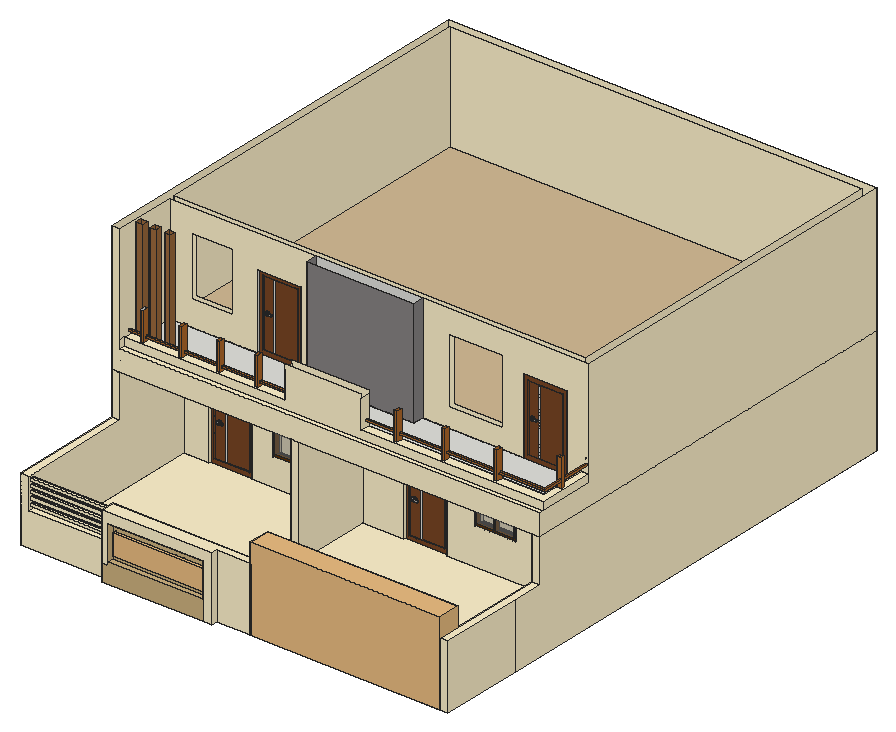
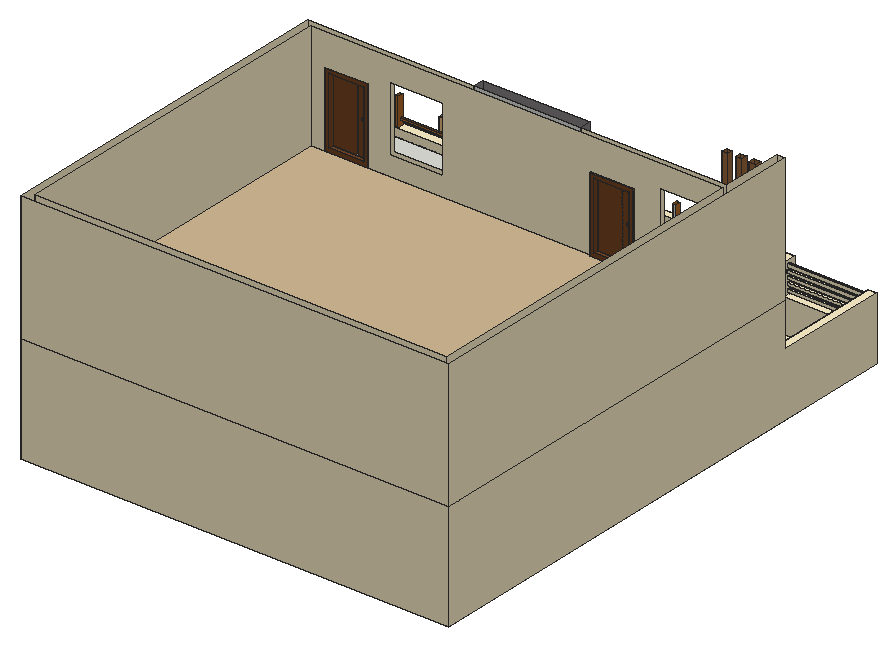
# SketchUp Ruby script. Lengths in inches.
U = 1.inch
M = Sketchup.active_model
def pt(a) = Geom::Point3d.new(a.map { |v| v * U })
def face(e, loops, mat)
  f = e.add_face(loops[0].map { |a| pt(a) })
  loops[1..].each { |l| e.add_face(l.map { |a| pt(a) }).erase! }
  f.material = f.back_material = mat if mat
  f
end
# faces: each face lists its corners as indices into pts; further lists are holes
def faces(e, pts, list, mat = nil) = list.each { |f| face(e, (f[0].is_a?(Array) ? f : [f]).map { |l| l.map { |i| pts[i] } }, mat) }
# xy, xz, yz: faces in a plane at the given z, y or x. An outline is a flat list of corners, or four numbers for a rectangle; further outlines are holes
def ring(l) = l.size == 4 ? [[l[0], l[1]], [l[2], l[1]], [l[2], l[3]], [l[0], l[3]]] : l.each_slice(2).to_a
def flat(e, list, mat, &to3) = list.each { |f| face(e, (f[0].is_a?(Array) ? f : [f]).map { |l| ring(l).map { |u, v| to3.(u, v) } }, mat) }
def xy(e, z, list, mat = nil) = flat(e, list, mat) { |x, y| [x, y, z] }
def xz(e, y, list, mat = nil) = flat(e, list, mat) { |x, z| [x, y, z] }
def yz(e, x, list, mat = nil) = flat(e, list, mat) { |y, z| [x, y, z] }
def lines(e, pts, list) = list.each { |a, b| e.add_line(pt(pts[a]), pt(pts[b])) }
# prism: a flat outline (further loops are holes) pulled along v
def prism(e, loops, v, mat = nil)
  f = face(e, loops, mat); d = Geom::Vector3d.new(v.map { |x| x * U })
  f.pushpull(f.normal.samedirection?(d) ? d.length : -d.length)
end
def box(e, o, s, mat = nil) = prism(e, [[o, [o[0] + s[0], o[1], o[2]], [o[0] + s[0], o[1] + s[1], o[2]], [o[0], o[1] + s[1], o[2]]]], [0, 0, s[2]], mat)
def at(x, y, z, deg = 0) = Geom::Transformation.translation(pt([x, y, z])) * Geom::Transformation.rotation(ORIGIN, Z_AXIS, deg.degrees)
def axes(o, x, y, z) = Geom::Transformation.new([*x, 0, *y, 0, *z, 0, *pt(o).to_a, 1])
def part(name) = M.definitions.add(name)
# library, detail: a bought-in or finely detailed component or shape, given as its bounding box
def library(name, o, s) = part(name).tap { |d| box(d.entities, o, s) }
def detail(e, o, s) = box(e.add_group.entities, o, s)
def put(e, d, t, mat = nil) = e.add_instance(d, t).tap { |i| i.material = mat if mat }
def group(e, t, mat = nil) = e.add_group.tap { |g| g.transformation = t; g.material = mat if mat }.entities
root = M.entities
M.materials.add("[Aluminum]").color = [179, 179, 179]
M.materials.add("[Brick Tumbled]").color = [135, 132, 132]
M.materials.add("[Color C08]").color = [102, 51, 0]
M.materials.add("[Color D01]").color = [255, 242, 204]
M.materials.add("[Formica Beige]").color = [211, 187, 149]
M.materials.add("[Stone Sandstone Ashlar Light]").color = [206, 178, 128]
M.materials.add("[Translucent Glass Gray]").color = [128, 128, 128]
M.materials["[Translucent Glass Gray]"].alpha = 0.5
M.materials.add("[Wood Bamboo]").color = [177, 105, 43]
M.materials.add("[Wood Floor]").color = [155, 105, 61]
M.materials.add("[Wood Veneer 01]").color = [120, 70, 37]
c1 = library("Wrought-iron gates",[-30,-13,0],[261.35,24.4,62.45])
c2 = part("Group\#1")
xy(c2.entities,0,[[0,1.5625,48,2.9375],[0,2.9375,48,11.9375]],"[Wood Veneer 01]")
xy(c2.entities,4.26,[[4.26,1.5625,43.74,2.9375],[4.26,2.9375,43.74,11.9375]],"[Wood Veneer 01]")
xy(c2.entities,41.66,[[8.83,0,8.83,1.4375,9.58,1.4375,9.58,0.72,15.08,0.72,15.08,0]],"[Aluminum]")
xy(c2.entities,43.35,[[8.83,0,15.08,0,15.08,0.72,9.58,0.72,9.58,1.4375,8.83,1.4375]],"[Aluminum]")
xy(c2.entities,79.74,[[4.26,1.5625,16.16,2.9375],[16.16,1.5625,16.99,2.9375],[16.99,1.5625,43.74,2.9375],[4.26,2.9375,43.74,11.9375]],"[Wood Veneer 01]")
xy(c2.entities,84,[[0,1.5625,48,2.9375],[0,2.9375,48,11.9375]],"[Wood Veneer 01]")
xz(c2.entities,0,[[8.83,41.66,15.08,43.35]],"[Aluminum]")
xz(c2.entities,0.72,[[9.58,41.66,15.08,43.35]],"[Aluminum]")
xz(c2.entities,1.4375,[[[9.24,40.44,9.77,40.51,10.27,40.72,10.7,41.05,11.03,41.47,11.23,41.97,11.3,42.5,11.23,43.04,11.03,43.54,10.7,43.96,10.27,44.29,9.77,44.5,9.24,44.57,8.71,44.5,8.21,44.29,7.78,43.96,7.45,43.54,7.25,43.04,7.18,42.5,7.25,41.97,7.45,41.47,7.78,41.05,8.21,40.72,8.71,40.51],[8.83,41.66,9.58,43.35]]],"[Aluminum]")
xz(c2.entities,1.5625,[[[0,0,48,84],[4.26,4.26,43.74,79.74]]],"[Wood Veneer 01]")
xz(c2.entities,2.9375,[[[0,0,48,84],[4.26,4.26,43.74,79.74]],[16.16,4.26,16.99,79.74]])
xz(c2.entities,2.9375,[[[4.26,4.26,16.16,79.74],[9.24,40.44,8.71,40.51,8.21,40.72,7.78,41.05,7.45,41.47,7.25,41.97,7.18,42.5,7.25,43.04,7.45,43.54,7.78,43.96,8.21,44.29,8.71,44.5,9.24,44.57,9.77,44.5,10.27,44.29,10.7,43.96,11.03,43.54,11.23,43.04,11.3,42.5,11.23,41.97,11.03,41.47,10.7,41.05,10.27,40.72,9.77,40.51]],[16.99,4.26,43.74,79.74]],"[Wood Veneer 01]")
xz(c2.entities,11.9375,[[[0,0,48,84],[4.26,4.26,43.74,79.74]]],"[Wood Veneer 01]")
yz(c2.entities,0,[[1.5625,0,2.9375,84],[2.9375,0,11.9375,84]],"[Wood Veneer 01]")
yz(c2.entities,4.26,[[1.5625,4.26,2.9375,79.74],[2.9375,4.26,11.9375,79.74]],"[Wood Veneer 01]")
yz(c2.entities,8.83,[[0,41.66,1.4375,43.35]],"[Aluminum]")
yz(c2.entities,9.58,[[0.72,41.66,1.4375,43.35]],"[Aluminum]")
yz(c2.entities,15.08,[[0,41.66,0.72,43.35]],"[Aluminum]")
yz(c2.entities,43.74,[[1.5625,4.26,2.9375,79.74],[2.9375,4.26,11.9375,79.74]],"[Wood Veneer 01]")
yz(c2.entities,48,[[1.5625,0,2.9375,84],[2.9375,0,11.9375,84]],"[Wood Veneer 01]")
p = [[8.71,2.9375,40.51],[9.24,2.9375,40.44],[9.24,1.4375,40.44],[8.71,1.4375,40.51],[9.77,2.9375,40.51],[9.77,1.4375,40.51],
  [8.21,2.9375,40.72],[8.21,1.4375,40.72],[10.27,2.9375,40.72],[10.27,1.4375,40.72],[7.78,2.9375,41.05],[7.78,1.4375,41.05],
  [10.7,2.9375,41.05],[10.7,1.4375,41.05],[7.45,2.9375,41.47],[7.45,1.4375,41.47],[11.03,2.9375,41.47],[11.03,1.4375,41.47],
  [7.25,2.9375,41.97],[7.25,1.4375,41.97],[11.23,2.9375,41.97],[11.23,1.4375,41.97],[7.18,2.9375,42.5],[7.18,1.4375,42.5],
  [11.3,2.9375,42.5],[11.3,1.4375,42.5],[7.25,2.9375,43.04],[7.25,1.4375,43.04],[11.23,2.9375,43.04],[11.23,1.4375,43.04],
  [7.45,2.9375,43.54],[7.45,1.4375,43.54],[11.03,2.9375,43.54],[11.03,1.4375,43.54],[7.78,2.9375,43.96],[7.78,1.4375,43.96],
  [10.7,2.9375,43.96],[10.7,1.4375,43.96],[8.21,2.9375,44.29],[8.21,1.4375,44.29],[10.27,2.9375,44.29],[10.27,1.4375,44.29],
  [8.71,2.9375,44.5],[8.71,1.4375,44.5],[9.77,2.9375,44.5],[9.77,1.4375,44.5],[9.24,2.9375,44.57],[9.24,1.4375,44.57]]
faces(c2.entities,p,[[0,1,2,3],[1,4,5,2],[6,0,3,7],[4,8,9,5],[10,6,7,11],[8,12,13,9],[14,10,11,15],[12,16,17,13],
  [18,14,15,19],[16,20,21,17],[22,18,19,23],[20,24,25,21],[26,22,23,27],[24,28,29,25],[30,26,27,31],[28,32,33,29],
  [34,30,31,35],[32,36,37,33],[38,34,35,39],[36,40,41,37],[42,38,39,43],[40,44,45,41],[46,42,43,47],[44,46,47,45]],"[Aluminum]")
c3 = library("RAMA",[0.59,0,0],[102.88,23.44,4])
c4 = part("Group\#4")
xy(c4.entities,0,[[0,0,52.875,9]],"[Color C08]")
xy(c4.entities,2.31,[[2.31,0,24.96,9],[26.98,0,50.56,9]],"[Color C08]")
xy(c4.entities,50.56,[[2.31,0,24.96,9],[26.98,0,50.56,9]],"[Color C08]")
xy(c4.entities,52.875,[[0,0,52.875,9]],"[Color C08]")
xz(c4.entities,0,[[[0,0,52.875,52.875],[26.98,2.31,50.56,50.56],[2.31,2.31,24.96,50.56]]],"[Color C08]")
xz(c4.entities,0,[[2.31,2.31,24.96,50.56],[26.98,2.31,50.56,50.56]],"[Translucent Glass Gray]")
xz(c4.entities,9,[[[0,0,52.875,52.875],[26.98,2.31,50.56,50.56],[2.31,2.31,24.96,50.56]]],"[Color C08]")
yz(c4.entities,0,[[0,0,9,52.875]],"[Color C08]")
yz(c4.entities,2.31,[[0,2.31,9,50.56]],"[Color C08]")
yz(c4.entities,24.96,[[0,2.31,9,50.56]],"[Color C08]")
yz(c4.entities,26.98,[[0,2.31,9,50.56]],"[Color C08]")
yz(c4.entities,50.56,[[0,2.31,9,50.56]],"[Color C08]")
yz(c4.entities,52.875,[[0,0,9,52.875]],"[Color C08]")
xy(root,0,[[96.6875,0,210.23,6.75],[210.23,0,220.17,6.75],[258.29,6.75,471,15.75],[9,15.75,471,15.75,471,225.0625,303.9375,225.0625,303.9375,235.3125,255.9375,235.3125,255.9375,225.0625,209.375,225.0625,209.375,135.4,200.375,135.4,200.375,225.0625,85.29,225.0625,85.29,235.3125,200.375,235.3125,200.375,597.75,9,597.75,9,235.3125,37.29,235.3125,37.29,225.0625,9,225.0625],[0,101.375,0,606.75,480,606.75,480,101.375,471,101.375,471,225.0625,303.9375,225.0625,303.9375,235.3125,471,235.3125,471,597.75,9,597.75,9,235.3125,37.29,235.3125,37.29,225.0625,9,225.0625,9,101.375],
  [200.375,135.4,209.375,235.3125],[85.29,225.0625,85.29,235.3125,200.375,235.3125,200.375,314.26,209.375,314.26,209.375,235.3125,200.375,235.3125,200.375,225.0625],[209.375,225.0625,255.9375,235.3125],[209.375,235.3125,471,235.3125,471,597.75,209.375,597.75,209.375,383.08,200.375,383.08,200.375,314.26,209.375,314.26],[200.375,383.08,209.375,597.75]],"[Color D01]")
xy(root,22.14,[[104,0,210.23,6.75]],"[Stone Sandstone Ashlar Light]")
xy(root,30.78,[[109.26,225.0625,164.32,235.3125]],"[Color D01]")
xy(root,37.75,[[9,6.75,96.6875,15.75]],"[Color D01]")
xy(root,40.97,[[9,8.99,96.6875,11.93]],"[Color D01]")
xy(root,41.23,[[335.7,225.0625,380.95,235.3125]],"[Color D01]")
xy(root,44.41,[[9,8.99,96.6875,11.93]],"[Color D01]")
xy(root,47.79,[[9,8.99,96.9375,11.93]],"[Color D01]")
xy(root,51.22,[[9,8.99,96.9375,11.93]],"[Color D01]")
xy(root,53.97,[[9,8.99,96.6875,11.93]],"[Color D01]")
xy(root,57.41,[[9,8.99,96.6875,11.93]],"[Color D01]")
xy(root,60.1,[[9,8.99,96,11.93]],"[Color D01]")
xy(root,61.125,[[104,0,210.23,6.75]],"[Stone Sandstone Ashlar Light]")
xy(root,63.54,[[9,8.99,96,11.93]],"[Color D01]")
xy(root,66.35,[[9,8.99,97.4375,11.93]],"[Color D01]")
xy(root,69.79,[[9,8.99,97.4375,11.93]],"[Color D01]")
xy(root,72,[[96.6875,0,220.17,0,220.17,6.75,258.29,6.75,258.29,15.75,96.6875,15.75],[0,6.75,9,135.4],[471,6.75,480,135.4]],"[Color D01]")
xy(root,84,[[37.29,225.0625,85.29,235.3125],[255.9375,225.0625,303.9375,235.3125]],"[Color D01]")
xy(root,94.1,[[335.7,225.0625,380.95,235.3125]],"[Color D01]")
xy(root,98.875,[[200.375,314.26,209.375,383.08]],"[Color D01]")
xy(root,102.59,[[109.26,225.0625,164.32,235.3125]],"[Color D01]")
xy(root,120,[[0,135.4,480,606.75]])
xy(root,120,[[0,135.4,9,135.4,9,225.0625,200.375,225.0625,200.375,135.4,209.375,135.4,209.375,597.75,200.375,597.75,200.375,235.3125,9,235.3125,9,597.75,471,597.75,471,235.3125,209.375,235.3125,209.375,225.0625,471,225.0625,471,135.4,480,135.4,480,606.75,0,606.75],[9,235.3125,200.375,597.75],[209.375,235.3125,471,597.75]],"[Color D01]")
xy(root,133,[[9,151.78,9,204.4,108.75,204.4,108.75,210.4,156.75,210.4,156.75,204.4,172.75,204.4,172.75,192.4,292.75,192.4,292.75,204.4,407.0625,204.4,407.0625,210.4,455.0625,210.4,455.0625,204.4,471,204.4,471,151.78]])
xy(root,143.9375,[[9,140.9,9,151.78,471,151.78,471,204.4,480,204.4,480,140.9],[[9,151.78,471,151.78,471,204.4,455.0625,204.4,455.0625,210.4,407.0625,210.4,407.0625,204.4,292.75,204.4,292.75,192.4,172.75,192.4,172.75,204.4,156.75,204.4,156.75,210.4,108.75,210.4,108.75,204.4,9,204.4],[11.75,154.17,19.6875,160.61],[27.8125,154.17,35,160.61],[43.5625,154.17,50.1875,160.61]],[172.75,192.4,292.75,204.4],[156.75,204.4,407.0625,210.4]])
xy(root,143.9375,[[9,135.4,480,140.9]],"[Color D01]")
xy(root,143.9375,[[9,210.4,471,597.75]],"[Formica Beige]")
xy(root,152.9375,[[[9,140.9,188.91,151.78],[25.45,143.88,28.82,150.13],[68.13,143.88,71.51,150.13],[110.26,143.88,113.63,150.13],[152.95,143.88,156.32,150.13]],[[274.98,140.9,480,140.9,480,204.4,471,204.4,471,151.78,274.98,151.78],[309.7,143.88,313.07,150.13],[362.95,143.88,366.32,150.13],[421.51,143.88,424.88,150.13],[472.3125,168.86,477.25,172.24]]],"[Color D01]")
xy(root,157.15,[[9,146.22,28.82,148.34]])
xy(root,157.15,[[28.82,146.22,188.91,148.34]],"[Wood Bamboo]")
xy(root,159.27,[[9,146.22,28.82,148.34],[28.82,146.22,188.91,148.34]],"[Wood Bamboo]")
xy(root,160.11,[[274.98,145.89,274.98,148.02,475.1875,148.02,475.1875,207.71,477.01,207.71,477.01,145.89]],"[Wood Bamboo]")
xz(root,0,[[210.23,0,220.17,0,220.17,72,96.6875,72,96.6875,18.4375,104,18.4375,104,61.125,210.23,61.125]],"[Color D01]")
xz(root,0,[[96.6875,0,210.23,0,210.23,22.14,104,22.14,104,18.4375,96.6875,18.4375]],"[Stone Sandstone Ashlar Light]")
xz(root,6.75,[[0,0,96.6875,0,96.6875,37.75,9,37.75,9,72,0,72],[220.17,0,258.29,0,258.29,72,220.25,72,220.25,61.125,220.17,61.125],[471,0,480,72],[220.17,61.125,220.25,72]],"[Color D01]")
xz(root,6.75,[[104,22.14,210.23,61.125]],"[Stone Sandstone Ashlar Light]")
xz(root,8.99,[[9,40.97,96.6875,44.41],[9,47.79,96.9375,51.22],[9,53.97,96.6875,57.41],[9,60.1,96,63.54],[9,66.35,97.4375,69.79]],"[Color D01]")
xz(root,11.93,[[9,40.97,96.6875,44.41],[9,47.79,96.9375,51.22],[9,53.97,96.6875,57.41],[9,60.1,96,63.54],[9,66.35,97.4375,69.79]],"[Color D01]")
xz(root,15.75,[[9,0,9,37.75,96.6875,37.75,96.6875,72,258.29,72,258.29,0]],"[Color D01]")
xz(root,135.4,[[200.375,0,209.375,120],[0,72,9,120],[471,72,480,120],[0,120,480,120,480,143.9375,9,143.9375,9,263.9375,0,263.9375]],"[Color D01]")
xz(root,140.9,[[9,143.9375,480,143.9375,480,152.9375,274.98,152.9375,274.98,188.9375,188.91,188.9375,188.91,152.9375,9,152.9375]],"[Color D01]")
xz(root,143.88,[[25.45,152.9375,28.82,185],[68.13,152.9375,71.51,184.18],[110.26,152.9375,113.63,184.18],[152.95,152.9375,156.32,184.4375],[309.7,152.9375,313.07,184],
  [362.95,152.9375,366.32,184.5625],[421.51,152.9375,424.88,184.18]],"[Wood Bamboo]")
xz(root,145.89,[[274.98,160.11,477.01,162.24]],"[Wood Bamboo]")
xz(root,146.22,[[9,157.15,28.82,159.27],[28.82,157.15,188.91,159.27]],"[Wood Bamboo]")
xz(root,148.02,[[274.98,160.11,475.1875,162.24]],"[Wood Bamboo]")
xz(root,148.34,[[9,157.15,28.82,159.27],[28.82,157.15,188.91,159.27]],"[Wood Bamboo]")
xz(root,150.13,[[110.26,152.9375,113.63,184.18],[152.95,152.9375,156.32,184.4375]])
xz(root,150.13,[[25.45,152.9375,28.82,185],[68.13,152.9375,71.51,184.18],[309.7,152.9375,313.07,184],[362.95,152.9375,366.32,184.5625],[421.51,152.9375,424.88,184.18]],"[Wood Bamboo]")
xz(root,151.78,[[9,133,471,143.9375]])
xz(root,151.78,[[9,143.9375,9,152.9375,188.91,152.9375,188.91,188.9375,274.98,188.9375,274.98,152.9375,471,152.9375,471,143.9375]],"[Color D01]")
xz(root,154.17,[[11.75,143.9375,19.6875,263.9375],[27.8125,143.9375,35,263.9375],[43.5625,143.9375,50.1875,263.9375]],"[Wood Floor]")
xz(root,160.61,[[11.75,143.9375,19.6875,263.9375],[27.8125,143.9375,35,263.9375],[43.5625,143.9375,50.1875,263.9375]],"[Wood Floor]")
xz(root,168.86,[[472.3125,152.9375,477.25,184.1875]],"[Wood Bamboo]")
xz(root,172.24,[[472.3125,152.9375,477.25,184.1875]],"[Wood Bamboo]")
xz(root,192.4,[[172.75,133,292.75,143.9375]])
xz(root,192.4,[[172.75,143.9375,292.75,263.9375]],"[Brick Tumbled]")
xz(root,204.4,[[9,133,108.75,143.9375],[156.75,133,172.75,143.9375],[292.75,133,407.0625,143.9375],[455.0625,133,471,143.9375],[172.75,143.9375,292.75,263.9375],
  [471,143.9375,480,152.9375]])
xz(root,204.4,[[[9,143.9375,108.75,143.9375,108.75,227.9375,156.75,227.9375,156.75,143.9375,172.75,143.9375,172.75,263.9375,9,263.9375],[33.82,172.75,80.13,238.56]],[[292.75,143.9375,407.0625,143.9375,407.0625,227.9375,455.0625,227.9375,455.0625,143.9375,471,143.9375,471,152.9375,480,152.9375,480,263.9375,292.75,263.9375],[322.9,165.73,382.78,238.86],[475.1875,166.24,477.01,168.36]]],"[Color D01]")
xz(root,207.71,[[475.1875,160.11,477.01,162.24]])
xz(root,210.4,[[108.75,133,156.75,143.9375],[407.0625,133,455.0625,143.9375]])
xz(root,210.4,[[[9,143.9375,9,263.9375,471,263.9375,471,143.9375,455.0625,143.9375,455.0625,227.9375,407.0625,227.9375,407.0625,143.9375,156.75,143.9375,156.75,227.9375,108.75,227.9375,108.75,143.9375],[322.9,165.73,382.78,238.86],[33.82,172.75,80.13,238.56]]],"[Color D01]")
xz(root,225.0625,[[[9,0,37.29,0,37.29,84,85.29,84,85.29,0,200.375,0,200.375,120,9,120],[109.26,30.78,164.32,102.59]],[[209.375,0,255.9375,0,255.9375,84,303.9375,84,303.9375,0,471,0,471,120,209.375,120],[335.7,41.23,380.95,94.1]]],"[Color D01]")
xz(root,235.3125,[[[9,0,9,120,200.375,120,200.375,0,85.29,0,85.29,84,37.29,84,37.29,0],[109.26,30.78,164.32,102.59]],[[209.375,0,209.375,120,471,120,471,0,303.9375,0,303.9375,84,255.9375,84,255.9375,0],[335.7,41.23,380.95,94.1]]],"[Color D01]")
xz(root,314.26,[[200.375,0,209.375,98.875]],"[Color D01]")
xz(root,383.08,[[200.375,0,209.375,98.875]],"[Color D01]")
xz(root,597.75,[[9,0,200.375,120],[200.375,0,209.375,120],[209.375,0,471,120],[9,143.9375,471,263.9375]],"[Color D01]")
xz(root,606.75,[[0,0,480,120],[0,120,480,263.9375]],"[Color D01]")
yz(root,0,[[6.75,0,6.75,72,135.4,72,135.4,120,606.75,120,606.75,0],[135.4,120,606.75,263.9375]],"[Color D01]")
yz(root,9,[[151.78,133,204.4,143.9375],[140.9,143.9375,151.78,152.9375]])
yz(root,9,[[[15.75,0,225.0625,0,225.0625,120,135.4,120,135.4,72,6.75,72,6.75,37.75,15.75,37.75],[8.99,40.97,11.93,44.41],[8.99,47.79,11.93,51.22],[8.99,53.97,11.93,57.41],[8.99,60.1,11.93,63.54],[8.99,66.35,11.93,69.79]],[235.3125,0,597.75,120],[135.4,143.9375,140.9,152.9375],[[151.78,143.9375,204.4,143.9375,204.4,263.9375,135.4,263.9375,135.4,152.9375,151.78,152.9375],[146.02,178.55,148.14,180.67],[146.02,171.67,148.14,173.8],[146.02,164.48,148.14,166.61],[146.22,157.15,148.34,159.27]],[210.4,143.9375,597.75,263.9375]],"[Color D01]")
yz(root,11.75,[[154.17,143.9375,160.61,263.9375]],"[Wood Floor]")
yz(root,19.6875,[[154.17,143.9375,160.61,263.9375]],"[Wood Floor]")
yz(root,25.45,[[143.88,152.9375,150.13,185]])
yz(root,27.8125,[[154.17,143.9375,160.61,263.9375]],"[Wood Floor]")
yz(root,28.82,[[146.22,157.15,148.34,159.27]])
yz(root,28.82,[[[143.88,152.9375,150.13,185],[146.02,178.55,148.14,180.67],[146.02,171.67,148.14,173.8],[146.02,164.48,148.14,166.61],[146.22,157.15,148.34,159.27]]],"[Wood Bamboo]")
yz(root,35,[[154.17,143.9375,160.61,263.9375]],"[Wood Floor]")
yz(root,37.29,[[225.0625,0,235.3125,84]],"[Color D01]")
yz(root,43.5625,[[154.17,143.9375,160.61,263.9375]],"[Wood Floor]")
yz(root,50.1875,[[154.17,143.9375,160.61,263.9375]],"[Wood Floor]")
yz(root,68.13,[[143.88,152.9375,150.13,184.18]],"[Wood Bamboo]")
yz(root,71.51,[[143.88,152.9375,150.13,184.18]],"[Wood Bamboo]")
yz(root,85.29,[[225.0625,0,235.3125,84]],"[Color D01]")
yz(root,96,[[8.99,60.1,11.93,63.54]],"[Color D01]")
yz(root,96.6875,[[[0,0,0,72,15.75,72,15.75,37.75,6.75,37.75,6.75,0],[8.99,40.97,11.93,44.41],[8.99,53.97,11.93,57.41]]],"[Color D01]")
yz(root,96.9375,[[8.99,47.79,11.93,51.22]],"[Color D01]")
yz(root,97.4375,[[8.99,66.35,11.93,69.79]],"[Color D01]")
yz(root,104,[[0,22.14,6.75,61.125]],"[Stone Sandstone Ashlar Light]")
yz(root,108.75,[[204.4,133,210.4,143.9375],[204.4,143.9375,210.4,227.9375]])
yz(root,109.26,[[225.0625,30.78,235.3125,102.59]],"[Color D01]")
yz(root,110.26,[[143.88,152.9375,150.13,184.18]],"[Wood Bamboo]")
yz(root,113.63,[[143.88,152.9375,150.13,184.18]],"[Wood Bamboo]")
yz(root,152.95,[[143.88,152.9375,150.13,184.4375]],"[Wood Bamboo]")
yz(root,156.32,[[143.88,152.9375,150.13,184.4375]],"[Wood Bamboo]")
yz(root,156.75,[[204.4,133,210.4,143.9375],[204.4,143.9375,210.4,227.9375]])
yz(root,164.32,[[225.0625,30.78,235.3125,102.59]],"[Color D01]")
yz(root,172.75,[[192.4,133,204.4,143.9375]])
yz(root,172.75,[[192.4,143.9375,204.4,263.9375]],"[Brick Tumbled]")
yz(root,188.91,[[[140.9,152.9375,151.78,184.18],[146.22,157.15,148.34,159.27]]],"[Color D01]")
yz(root,200.375,[[135.4,0,225.0625,120],[235.3125,0,235.3125,120,597.75,120,597.75,0,383.08,0,383.08,98.875,314.26,98.875,314.26,0]],"[Color D01]")
yz(root,209.375,[[135.4,0,225.0625,120],[225.0625,0,235.3125,120],[235.3125,0,314.26,0,314.26,98.875,383.08,98.875,383.08,0,597.75,0,597.75,120,235.3125,120]],"[Color D01]")
yz(root,210.23,[[0,22.14,6.75,61.125]],"[Stone Sandstone Ashlar Light]")
yz(root,220.17,[[0,0,6.75,72]],"[Color D01]")
yz(root,255.9375,[[225.0625,0,235.3125,84]],"[Color D01]")
yz(root,258.29,[[6.75,0,15.75,72]],"[Color D01]")
yz(root,274.98,[[[140.9,152.9375,151.78,184.18],[145.89,177.99,148.02,180.49],[145.89,172.43,148.02,174.55],[145.89,166.24,148.02,168.36],[145.89,160.11,148.02,162.24]]],"[Color D01]")
yz(root,292.75,[[192.4,133,204.4,143.9375]])
yz(root,292.75,[[192.4,143.9375,204.4,263.9375]],"[Brick Tumbled]")
yz(root,303.9375,[[225.0625,0,235.3125,84]],"[Color D01]")
yz(root,309.7,[[143.88,152.9375,150.13,184]],"[Wood Bamboo]")
yz(root,313.07,[[143.88,152.9375,150.13,184]],"[Wood Bamboo]")
yz(root,335.7,[[225.0625,41.23,235.3125,94.1]],"[Color D01]")
yz(root,362.95,[[143.88,152.9375,150.13,184.5625]],"[Wood Bamboo]")
yz(root,366.32,[[143.88,152.9375,150.13,184.5625]],"[Wood Bamboo]")
yz(root,380.95,[[225.0625,41.23,235.3125,94.1]],"[Color D01]")
yz(root,407.0625,[[204.4,133,210.4,143.9375],[204.4,143.9375,210.4,227.9375]])
yz(root,421.51,[[143.88,152.9375,150.13,184.18]],"[Wood Bamboo]")
yz(root,424.88,[[143.88,152.9375,150.13,184.18]],"[Wood Bamboo]")
yz(root,455.0625,[[204.4,133,210.4,143.9375],[204.4,143.9375,210.4,227.9375]])
yz(root,471,[[151.78,133,204.4,143.9375]])
yz(root,471,[[6.75,0,6.75,72,135.4,72,135.4,120,225.0625,120,225.0625,0],[235.3125,0,597.75,120],[151.78,143.9375,204.4,152.9375],[210.4,143.9375,597.75,263.9375]],"[Color D01]")
yz(root,472.3125,[[168.86,152.9375,172.24,184.1875]],"[Wood Bamboo]")
yz(root,475.1875,[[148.02,160.11,207.71,162.24]],"[Wood Bamboo]")
yz(root,477.01,[[145.89,160.11,207.71,162.24]],"[Wood Bamboo]")
yz(root,477.25,[[168.86,152.9375,172.24,184.1875]],"[Wood Bamboo]")
yz(root,480,[[6.75,0,101.375,72],[101.375,0,606.75,0,606.75,120,135.4,120,135.4,72,101.375,72],[135.4,120,606.75,120,606.75,263.9375,204.4,263.9375,204.4,143.9375,135.4,143.9375],[140.9,143.9375,204.4,152.9375]],"[Color D01]")
p = [[1102.375,144.4,120],[1102.375,144.4,132],[209.375,225.0625,0],[209.375,225.0625,-6.25],[9,597.75,131.9375],[9,597.75,143.9375],
  [9,204.4,131.9375],[9,204.4,133],[471,204.4,131.9375],[471,204.4,133],[9,144.4,131.9375],[9,135.4,131.9375],
  [9,210.4,131.9375],[9,210.4,143.9375],[9,144.4,143.9375],[471,597.75,131.9375],[471,597.75,143.9375],[471,210.4,131.9375],
  [471,210.4,143.9375]]
lines(root,p,[[0,1],[2,3],[4,5],[6,7],[8,9],[10,11],[12,13],[10,14],[15,16],[17,18]])
put(root,c1,axes([282.61,19.43,0],[0.81431,0,0],[0,1,0],[0,0,1.5]))
put(root,c2,at(37.29,225.0625,0))
put(root,c2,at(255.9375,225.0625,0))
put(root,c3,axes([106.05,6.75,27.75],[1,0,0],[0,0,1],[0,-1,0]))
put(root,c4,axes([108.89,225.0625,30.78],[1.0483,0,0],[0,0.5,0],[0,0,1.35816]))
put(root,c4,axes([335.14,225.0625,41.23],[0.86636,0,0],[0,0.5,0],[0,0,1]))
g1 = group(root,at(407.0625,202.84,143.9375))
xy(g1,0,[[0,1.02,48,1.91],[0,1.91,48,7.76]],"[Wood Veneer 01]")
xy(g1,4.26,[[4.26,1.02,43.74,1.91],[4.26,1.91,43.74,7.76]],"[Wood Veneer 01]")
xy(g1,41.66,[[8.83,0,8.83,0.93,9.58,0.93,9.58,0.47,15.08,0.47,15.08,0]],"[Aluminum]")
xy(g1,43.35,[[8.83,0,15.08,0,15.08,0.47,9.58,0.47,9.58,0.93,8.83,0.93]],"[Aluminum]")
xy(g1,79.74,[[4.26,1.02,16.16,1.91],[16.16,1.02,16.99,1.91],[16.99,1.02,43.74,1.91],[4.26,1.91,43.74,7.76]],"[Wood Veneer 01]")
xy(g1,84,[[0,1.02,48,1.91],[0,1.91,48,7.76]],"[Wood Veneer 01]")
xz(g1,0,[[8.83,41.66,15.08,43.35]],"[Aluminum]")
xz(g1,0.47,[[9.58,41.66,15.08,43.35]],"[Aluminum]")
xz(g1,0.93,[[[9.24,40.44,9.77,40.51,10.27,40.72,10.7,41.05,11.03,41.47,11.23,41.97,11.3,42.5,11.23,43.04,11.03,43.54,10.7,43.96,10.27,44.29,9.77,44.5,9.24,44.57,8.71,44.5,8.21,44.29,7.78,43.96,7.45,43.54,7.25,43.04,7.18,42.5,7.25,41.97,7.45,41.47,7.78,41.05,8.21,40.72,8.71,40.51],[8.83,41.66,9.58,43.35]]],"[Aluminum]")
xz(g1,1.02,[[[0,0,48,84],[4.26,4.26,43.74,79.74]]],"[Wood Veneer 01]")
xz(g1,1.91,[[[0,0,48,84],[4.26,4.26,43.74,79.74]],[16.16,4.26,16.99,79.74]])
xz(g1,1.91,[[[4.26,4.26,16.16,79.74],[9.24,40.44,8.71,40.51,8.21,40.72,7.78,41.05,7.45,41.47,7.25,41.97,7.18,42.5,7.25,43.04,7.45,43.54,7.78,43.96,8.21,44.29,8.71,44.5,9.24,44.57,9.77,44.5,10.27,44.29,10.7,43.96,11.03,43.54,11.23,43.04,11.3,42.5,11.23,41.97,11.03,41.47,10.7,41.05,10.27,40.72,9.77,40.51]],[16.99,4.26,43.74,79.74]],"[Wood Veneer 01]")
xz(g1,7.76,[[[0,0,48,84],[4.26,4.26,43.74,79.74]]],"[Wood Veneer 01]")
yz(g1,0,[[1.02,0,1.91,84],[1.91,0,7.76,84]],"[Wood Veneer 01]")
yz(g1,4.26,[[1.02,4.26,1.91,79.74],[1.91,4.26,7.76,79.74]],"[Wood Veneer 01]")
yz(g1,8.83,[[0,41.66,0.93,43.35]],"[Aluminum]")
yz(g1,9.58,[[0.47,41.66,0.93,43.35]],"[Aluminum]")
yz(g1,15.08,[[0,41.66,0.47,43.35]],"[Aluminum]")
yz(g1,43.74,[[1.02,4.26,1.91,79.74],[1.91,4.26,7.76,79.74]],"[Wood Veneer 01]")
yz(g1,48,[[1.02,0,1.91,84],[1.91,0,7.76,84]],"[Wood Veneer 01]")
p = [[8.71,1.91,40.51],[9.24,1.91,40.44],[9.24,0.93,40.44],[8.71,0.93,40.51],[9.77,1.91,40.51],[9.77,0.93,40.51],
  [8.21,1.91,40.72],[8.21,0.93,40.72],[10.27,1.91,40.72],[10.27,0.93,40.72],[7.78,1.91,41.05],[7.78,0.93,41.05],
  [10.7,1.91,41.05],[10.7,0.93,41.05],[7.45,1.91,41.47],[7.45,0.93,41.47],[11.03,1.91,41.47],[11.03,0.93,41.47],
  [7.25,1.91,41.97],[7.25,0.93,41.97],[11.23,1.91,41.97],[11.23,0.93,41.97],[7.18,1.91,42.5],[7.18,0.93,42.5],
  [11.3,1.91,42.5],[11.3,0.93,42.5],[7.25,1.91,43.04],[7.25,0.93,43.04],[11.23,1.91,43.04],[11.23,0.93,43.04],
  [7.45,1.91,43.54],[7.45,0.93,43.54],[11.03,1.91,43.54],[11.03,0.93,43.54],[7.78,1.91,43.96],[7.78,0.93,43.96],
  [10.7,1.91,43.96],[10.7,0.93,43.96],[8.21,1.91,44.29],[8.21,0.93,44.29],[10.27,1.91,44.29],[10.27,0.93,44.29],
  [8.71,1.91,44.5],[8.71,0.93,44.5],[9.77,1.91,44.5],[9.77,0.93,44.5],[9.24,1.91,44.57],[9.24,0.93,44.57]]
faces(g1,p,[[0,1,2,3],[1,4,5,2],[6,0,3,7],[4,8,9,5],[10,6,7,11],[8,12,13,9],[14,10,11,15],[12,16,17,13],
  [18,14,15,19],[16,20,21,17],[22,18,19,23],[20,24,25,21],[26,22,23,27],[24,28,29,25],[30,26,27,31],[28,32,33,29],
  [34,30,31,35],[32,36,37,33],[38,34,35,39],[36,40,41,37],[42,38,39,43],[40,44,45,41],[46,42,43,47],[44,46,47,45]],"[Aluminum]")
put(root,c2,axes([108.75,204.4,143.9375],[1,0,0],[0,0.65,0],[0,0,1]))
